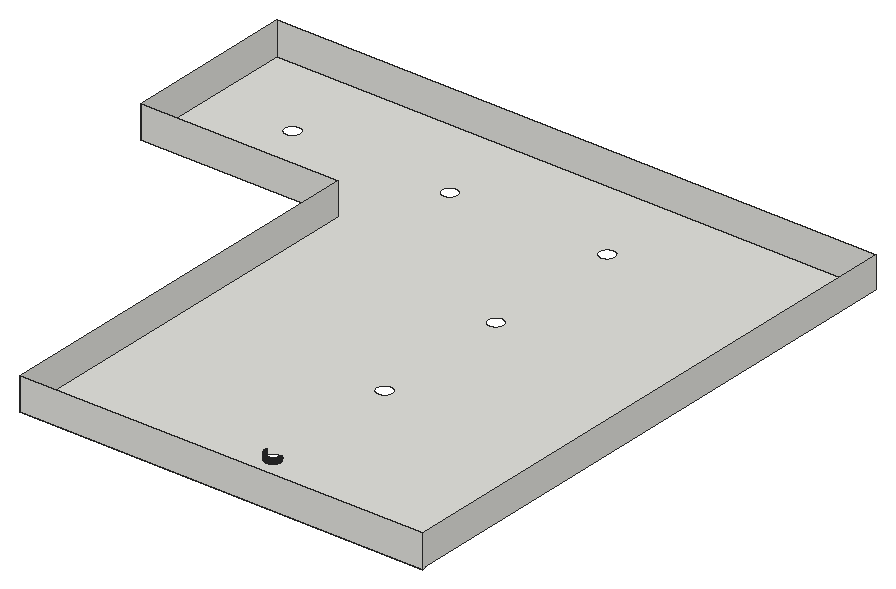
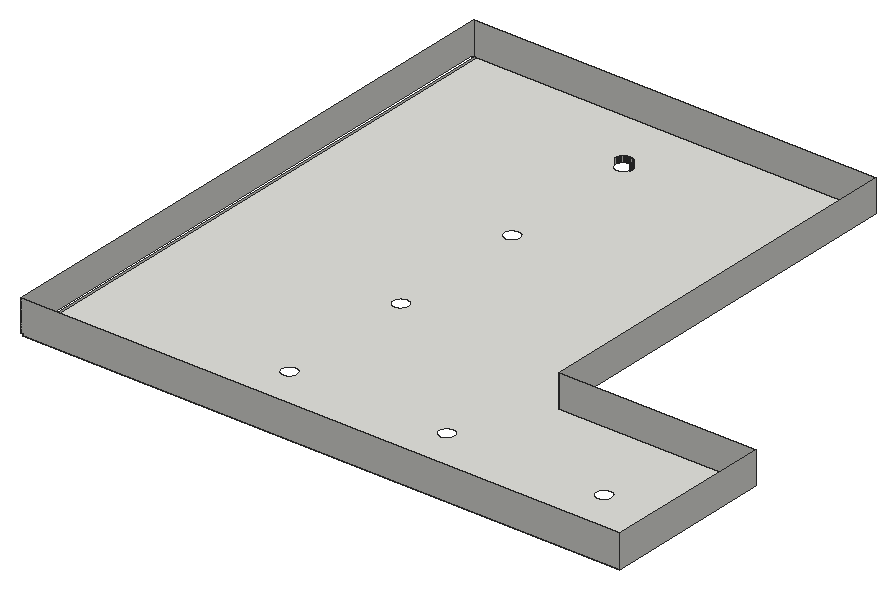
# SketchUp Ruby script. Lengths in inches.
U = 1.inch
M = Sketchup.active_model
def pt(a) = Geom::Point3d.new(a.map { |v| v * U })
def face(e, loops, mat)
  f = e.add_face(loops[0].map { |a| pt(a) })
  loops[1..].each { |l| e.add_face(l.map { |a| pt(a) }).erase! }
  f.material = f.back_material = mat if mat
  f
end
# faces: each face lists its corners as indices into pts; further lists are holes
def faces(e, pts, list, mat = nil) = list.each { |f| face(e, (f[0].is_a?(Array) ? f : [f]).map { |l| l.map { |i| pts[i] } }, mat) }
# xy, xz, yz: faces in a plane at the given z, y or x. An outline is a flat list of corners, or four numbers for a rectangle; further outlines are holes
def ring(l) = l.size == 4 ? [[l[0], l[1]], [l[2], l[1]], [l[2], l[3]], [l[0], l[3]]] : l.each_slice(2).to_a
def flat(e, list, mat, &to3) = list.each { |f| face(e, (f[0].is_a?(Array) ? f : [f]).map { |l| ring(l).map { |u, v| to3.(u, v) } }, mat) }
def xy(e, z, list, mat = nil) = flat(e, list, mat) { |x, y| [x, y, z] }
def xz(e, y, list, mat = nil) = flat(e, list, mat) { |x, z| [x, y, z] }
def yz(e, x, list, mat = nil) = flat(e, list, mat) { |y, z| [x, y, z] }
def lines(e, pts, list) = list.each { |a, b| e.add_line(pt(pts[a]), pt(pts[b])) }
# prism: a flat outline (further loops are holes) pulled along v
def prism(e, loops, v, mat = nil)
  f = face(e, loops, mat); d = Geom::Vector3d.new(v.map { |x| x * U })
  f.pushpull(f.normal.samedirection?(d) ? d.length : -d.length)
end
def box(e, o, s, mat = nil) = prism(e, [[o, [o[0] + s[0], o[1], o[2]], [o[0] + s[0], o[1] + s[1], o[2]], [o[0], o[1] + s[1], o[2]]]], [0, 0, s[2]], mat)
def at(x, y, z, deg = 0) = Geom::Transformation.translation(pt([x, y, z])) * Geom::Transformation.rotation(ORIGIN, Z_AXIS, deg.degrees)
def axes(o, x, y, z) = Geom::Transformation.new([*x, 0, *y, 0, *z, 0, *pt(o).to_a, 1])
def part(name) = M.definitions.add(name)
# library, detail: a bought-in or finely detailed component or shape, given as its bounding box
def library(name, o, s) = part(name).tap { |d| box(d.entities, o, s) }
def detail(e, o, s) = box(e.add_group.entities, o, s)
def put(e, d, t, mat = nil) = e.add_instance(d, t).tap { |i| i.material = mat if mat }
def group(e, t, mat = nil) = e.add_group.tap { |g| g.transformation = t; g.material = mat if mat }.entities
root = M.entities
xy(root,108,[[[82,0,82,147,9,147,9,210,230,210,230,1,231,1,231,0],[156.34,175.5,156.66,175.5,156.74,175.51,156.8125,175.52,156.89,175.53,157.05,175.55,157.125,175.57,157.2,175.58,157.28,175.6,157.35,175.625,157.43,175.65,157.5,175.67,157.58,175.7,157.79,175.79,157.86,175.83,157.93,175.86,158.07,175.94,158.13,175.98,158.2,176.03,158.26,176.07,158.33,176.12,158.57,176.32,158.62,176.38,158.68,176.43,158.88,176.67,158.93,176.74,158.97,176.8,159.02,176.87,159.06,176.93,159.14,177.07,159.17,177.14,159.21,177.21,159.3,177.42,159.33,177.5,159.35,177.57,159.375,177.65,159.4,177.72,159.42,177.8,159.43,177.875,159.45,177.95,159.47,178.11,159.48,178.1875,159.49,178.26,159.5,178.34,159.5,178.66,159.49,178.74,159.48,178.8125,159.47,178.89,159.45,179.05,159.43,179.125,159.42,179.2,159.4,179.28,159.375,179.35,159.35,179.43,159.33,179.5,159.3,179.58,159.21,179.79,159.17,179.86,159.14,179.93,159.06,180.07,159.02,180.13,158.97,180.2,158.93,180.26,158.88,180.33,158.68,180.57,158.62,180.62,158.57,180.68,158.33,180.88,158.26,180.93,158.2,180.97,158.13,181.02,158.07,181.06,157.93,181.14,157.86,181.17,157.79,181.21,157.58,181.3,157.5,181.33,157.43,181.35,157.35,181.375,157.28,181.4,157.2,181.42,157.125,181.43,157.05,181.45,156.89,181.47,156.8125,181.48,156.74,181.49,156.66,181.5,156.34,181.5,156.26,181.49,156.1875,181.48,156.11,181.47,155.95,181.45,155.875,181.43,155.8,181.42,155.72,181.4,155.65,181.375,155.57,181.35,155.5,181.33,155.42,181.3,155.21,181.21,155.14,181.17,155.07,181.14,154.93,181.06,154.87,181.02,154.8,180.97,154.74,180.93,154.67,180.88,154.43,180.68,154.38,180.62,154.32,180.57,154.12,180.33,154.07,180.26,154.03,180.2,153.98,180.13,153.94,180.07,153.86,179.93,153.83,179.86,153.79,179.79,153.7,179.58,153.67,179.5,153.65,179.43,153.625,179.35,153.6,179.28,153.58,179.2,153.57,179.125,153.55,179.05,153.53,178.89,153.52,178.8125,153.51,178.74,153.5,178.66,153.5,178.34,153.51,178.26,153.52,178.1875,153.53,178.11,153.55,177.95,153.57,177.875,153.58,177.8,153.6,177.72,153.625,177.65,153.65,177.57,153.67,177.5,153.7,177.42,153.79,177.21,153.83,177.14,153.86,177.07,153.94,176.93,153.98,176.87,154.03,176.8,154.07,176.74,154.12,176.67,154.32,176.43,154.38,176.38,154.43,176.32,154.67,176.12,154.74,176.07,154.8,176.03,154.87,175.98,154.93,175.94,155.07,175.86,155.14,175.83,155.21,175.79,155.42,175.7,155.5,175.67,155.57,175.65,155.65,175.625,155.72,175.6,155.8,175.58,155.875,175.57,155.95,175.55,156.11,175.53,156.1875,175.52,156.26,175.51],[156.34,124,156.66,124,156.74,124.01,156.8125,124.02,156.89,124.03,157.05,124.05,157.125,124.07,157.2,124.08,157.28,124.1,157.35,124.125,157.43,124.15,157.5,124.17,157.58,124.2,157.79,124.29,157.86,124.33,157.93,124.36,158.07,124.44,158.13,124.48,158.2,124.53,158.26,124.57,158.33,124.62,158.57,124.82,158.62,124.88,158.68,124.93,158.88,125.17,158.93,125.24,158.97,125.3,159.02,125.37,159.06,125.43,159.14,125.57,159.17,125.64,159.21,125.71,159.3,125.92,159.33,126,159.35,126.07,159.375,126.15,159.4,126.22,159.42,126.3,159.43,126.375,159.45,126.45,159.47,126.61,159.48,126.6875,159.49,126.76,159.5,126.84,159.5,127.16,159.49,127.24,159.48,127.3125,159.47,127.39,159.45,127.55,159.43,127.625,159.42,127.7,159.4,127.78,159.375,127.85,159.35,127.93,159.33,128,159.3,128.08,159.21,128.29,159.17,128.36,159.14,128.43,159.06,128.57,159.02,128.63,158.97,128.7,158.93,128.76,158.88,128.83,158.68,129.07,158.62,129.12,158.57,129.18,158.33,129.38,158.26,129.43,158.2,129.47,158.13,129.52,158.07,129.56,157.93,129.64,157.86,129.67,157.79,129.71,157.58,129.8,157.5,129.83,157.43,129.85,157.35,129.875,157.28,129.9,157.2,129.92,157.125,129.93,157.05,129.95,156.89,129.97,156.8125,129.98,156.74,129.99,156.66,130,156.34,130,156.26,129.99,156.1875,129.98,156.11,129.97,155.95,129.95,155.875,129.93,155.8,129.92,155.72,129.9,155.65,129.875,155.57,129.85,155.5,129.83,155.42,129.8,155.21,129.71,155.14,129.67,155.07,129.64,154.93,129.56,154.87,129.52,154.8,129.47,154.74,129.43,154.67,129.38,154.43,129.18,154.38,129.12,154.32,129.07,154.12,128.83,154.07,128.76,154.03,128.7,153.98,128.63,153.94,128.57,153.86,128.43,153.83,128.36,153.79,128.29,153.7,128.08,153.67,128,153.65,127.93,153.625,127.85,153.6,127.78,153.58,127.7,153.57,127.625,153.55,127.55,153.53,127.39,153.52,127.3125,153.51,127.24,153.5,127.16,153.5,126.84,153.51,126.76,153.52,126.6875,153.53,126.61,153.55,126.45,153.57,126.375,153.58,126.3,153.6,126.22,153.625,126.15,153.65,126.07,153.67,126,153.7,125.92,153.79,125.71,153.83,125.64,153.86,125.57,153.94,125.43,153.98,125.37,154.03,125.3,154.07,125.24,154.12,125.17,154.32,124.93,154.38,124.88,154.43,124.82,154.67,124.62,154.74,124.57,154.8,124.53,154.87,124.48,154.93,124.44,155.07,124.36,155.14,124.33,155.21,124.29,155.42,124.2,155.5,124.17,155.57,124.15,155.65,124.125,155.72,124.1,155.8,124.08,155.875,124.07,155.95,124.05,156.11,124.03,156.1875,124.02,156.26,124.01],[156.34,72.5,156.66,72.5,156.74,72.51,156.8125,72.52,156.89,72.53,157.05,72.55,157.125,72.57,157.2,72.58,157.28,72.6,157.35,72.625,157.43,72.65,157.5,72.67,157.58,72.7,157.79,72.79,157.86,72.83,157.93,72.86,158.07,72.94,158.13,72.98,158.2,73.03,158.26,73.07,158.33,73.12,158.57,73.32,158.62,73.38,158.68,73.43,158.88,73.67,158.93,73.74,158.97,73.8,159.02,73.87,159.06,73.93,159.14,74.07,159.17,74.14,159.21,74.21,159.3,74.42,159.33,74.5,159.35,74.57,159.375,74.65,159.4,74.72,159.42,74.8,159.43,74.875,159.45,74.95,159.47,75.11,159.48,75.1875,159.49,75.26,159.5,75.34,159.5,75.66,159.49,75.74,159.48,75.8125,159.47,75.89,159.45,76.05,159.43,76.125,159.42,76.2,159.4,76.28,159.375,76.35,159.35,76.43,159.33,76.5,159.3,76.58,159.21,76.79,159.17,76.86,159.14,76.93,159.06,77.07,159.02,77.13,158.97,77.2,158.93,77.26,158.88,77.33,158.68,77.57,158.62,77.62,158.57,77.68,158.33,77.88,158.26,77.93,158.2,77.97,158.13,78.02,158.07,78.06,157.93,78.14,157.86,78.17,157.79,78.21,157.58,78.3,157.5,78.33,157.43,78.35,157.35,78.375,157.28,78.4,157.2,78.42,157.125,78.43,157.05,78.45,156.89,78.47,156.8125,78.48,156.74,78.49,156.66,78.5,156.34,78.5,156.26,78.49,156.1875,78.48,156.11,78.47,155.95,78.45,155.875,78.43,155.8,78.42,155.72,78.4,155.65,78.375,155.57,78.35,155.5,78.33,155.42,78.3,155.21,78.21,155.14,78.17,155.07,78.14,154.93,78.06,154.87,78.02,154.8,77.97,154.74,77.93,154.67,77.88,154.43,77.68,154.38,77.62,154.32,77.57,154.12,77.33,154.07,77.26,154.03,77.2,153.98,77.13,153.94,77.07,153.86,76.93,153.83,76.86,153.79,76.79,153.7,76.58,153.67,76.5,153.65,76.43,153.625,76.35,153.6,76.28,153.58,76.2,153.57,76.125,153.55,76.05,153.53,75.89,153.52,75.8125,153.51,75.74,153.5,75.66,153.5,75.34,153.51,75.26,153.52,75.1875,153.53,75.11,153.55,74.95,153.57,74.875,153.58,74.8,153.6,74.72,153.625,74.65,153.65,74.57,153.67,74.5,153.7,74.42,153.79,74.21,153.83,74.14,153.86,74.07,153.94,73.93,153.98,73.87,154.03,73.8,154.07,73.74,154.12,73.67,154.32,73.43,154.38,73.38,154.43,73.32,154.67,73.12,154.74,73.07,154.8,73.03,154.87,72.98,154.93,72.94,155.07,72.86,155.14,72.83,155.21,72.79,155.42,72.7,155.5,72.67,155.57,72.65,155.65,72.625,155.72,72.6,155.8,72.58,155.875,72.57,155.95,72.55,156.11,72.53,156.1875,72.52,156.26,72.51],[156.34,21,156.66,21,156.74,21.01,156.8125,21.02,156.89,21.03,157.05,21.05,157.125,21.07,157.2,21.08,157.28,21.1,157.35,21.125,157.43,21.15,157.5,21.17,157.58,21.2,157.79,21.29,157.86,21.33,157.93,21.36,158.07,21.44,158.13,21.48,158.2,21.53,158.26,21.57,158.33,21.62,158.57,21.82,158.62,21.88,158.68,21.93,158.88,22.17,158.93,22.24,158.97,22.3,159.02,22.37,159.06,22.43,159.14,22.57,159.17,22.64,159.21,22.71,159.3,22.92,159.33,23,159.35,23.07,159.375,23.15,159.4,23.22,159.42,23.3,159.43,23.375,159.45,23.45,159.47,23.61,159.48,23.6875,159.49,23.76,159.5,23.84,159.5,24.16,159.49,24.24,159.48,24.3125,159.47,24.39,159.45,24.55,159.43,24.625,159.42,24.7,159.4,24.78,159.375,24.85,159.35,24.93,159.33,25,159.3,25.08,159.21,25.29,159.17,25.36,159.14,25.43,159.06,25.57,159.02,25.63,158.97,25.7,158.93,25.76,158.88,25.83,158.68,26.07,158.62,26.12,158.57,26.18,158.33,26.38,158.26,26.43,158.2,26.47,158.13,26.52,158.07,26.56,157.93,26.64,157.86,26.67,157.79,26.71,157.58,26.8,157.5,26.83,157.43,26.85,157.35,26.875,157.28,26.9,157.2,26.92,157.125,26.93,157.05,26.95,156.89,26.97,156.8125,26.98,156.74,26.99,156.66,27,156.34,27,156.26,26.99,156.1875,26.98,156.11,26.97,155.95,26.95,155.875,26.93,155.8,26.92,155.72,26.9,155.65,26.875,155.57,26.85,155.5,26.83,155.42,26.8,155.21,26.71,155.14,26.67,155.07,26.64,154.93,26.56,154.87,26.52,154.8,26.47,154.74,26.43,154.67,26.38,154.43,26.18,154.38,26.12,154.32,26.07,154.12,25.83,154.07,25.76,154.03,25.7,153.98,25.63,153.94,25.57,153.86,25.43,153.83,25.36,153.79,25.29,153.7,25.08,153.67,25,153.65,24.93,153.625,24.85,153.6,24.78,153.58,24.7,153.57,24.625,153.55,24.55,153.53,24.39,153.52,24.3125,153.51,24.24,153.5,24.16,153.5,23.84,153.51,23.76,153.52,23.6875,153.53,23.61,153.55,23.45,153.57,23.375,153.58,23.3,153.6,23.22,153.625,23.15,153.65,23.07,153.67,23,153.7,22.92,153.79,22.71,153.83,22.64,153.86,22.57,153.94,22.43,153.98,22.37,154.03,22.3,154.07,22.24,154.12,22.17,154.32,21.93,154.38,21.88,154.43,21.82,154.67,21.62,154.74,21.57,154.8,21.53,154.87,21.48,154.93,21.44,155.07,21.36,155.14,21.33,155.21,21.29,155.42,21.2,155.5,21.17,155.57,21.15,155.65,21.125,155.72,21.1,155.8,21.08,155.875,21.07,155.95,21.05,156.11,21.03,156.1875,21.02,156.26,21.01],[98.09,175.5,98.41,175.5,98.49,175.51,98.5625,175.52,98.64,175.53,98.8,175.55,98.875,175.57,98.95,175.58,99.03,175.6,99.1,175.625,99.18,175.65,99.25,175.67,99.33,175.7,99.54,175.79,99.61,175.83,99.68,175.86,99.82,175.94,99.88,175.98,99.95,176.03,100.01,176.07,100.08,176.12,100.32,176.32,100.37,176.38,100.43,176.43,100.63,176.67,100.68,176.74,100.72,176.8,100.77,176.87,100.81,176.93,100.89,177.07,100.92,177.14,100.96,177.21,101.05,177.42,101.08,177.5,101.1,177.57,101.125,177.65,101.15,177.72,101.17,177.8,101.18,177.875,101.2,177.95,101.22,178.11,101.23,178.1875,101.24,178.26,101.25,178.34,101.25,178.66,101.24,178.74,101.23,178.8125,101.22,178.89,101.2,179.05,101.18,179.125,101.17,179.2,101.15,179.28,101.125,179.35,101.1,179.43,101.08,179.5,101.05,179.58,100.96,179.79,100.92,179.86,100.89,179.93,100.81,180.07,100.77,180.13,100.72,180.2,100.68,180.26,100.63,180.33,100.43,180.57,100.37,180.62,100.32,180.68,100.08,180.88,100.01,180.93,99.95,180.97,99.88,181.02,99.82,181.06,99.68,181.14,99.61,181.17,99.54,181.21,99.33,181.3,99.25,181.33,99.18,181.35,99.1,181.375,99.03,181.4,98.95,181.42,98.875,181.43,98.8,181.45,98.64,181.47,98.5625,181.48,98.49,181.49,98.41,181.5,98.09,181.5,98.01,181.49,97.9375,181.48,97.86,181.47,97.7,181.45,97.625,181.43,97.55,181.42,97.47,181.4,97.4,181.375,97.32,181.35,97.25,181.33,97.17,181.3,96.96,181.21,96.89,181.17,96.82,181.14,96.68,181.06,96.62,181.02,96.55,180.97,96.49,180.93,96.42,180.88,96.18,180.68,96.13,180.62,96.07,180.57,95.87,180.33,95.82,180.26,95.78,180.2,95.73,180.13,95.69,180.07,95.61,179.93,95.58,179.86,95.54,179.79,95.45,179.58,95.42,179.5,95.4,179.43,95.375,179.35,95.35,179.28,95.33,179.2,95.32,179.125,95.3,179.05,95.28,178.89,95.27,178.8125,95.26,178.74,95.25,178.66,95.25,178.34,95.26,178.26,95.27,178.1875,95.28,178.11,95.3,177.95,95.32,177.875,95.33,177.8,95.35,177.72,95.375,177.65,95.4,177.57,95.42,177.5,95.45,177.42,95.54,177.21,95.58,177.14,95.61,177.07,95.69,176.93,95.73,176.87,95.78,176.8,95.82,176.74,95.87,176.67,96.07,176.43,96.13,176.38,96.18,176.32,96.42,176.12,96.49,176.07,96.55,176.03,96.62,175.98,96.68,175.94,96.82,175.86,96.89,175.83,96.96,175.79,97.17,175.7,97.25,175.67,97.32,175.65,97.4,175.625,97.47,175.6,97.55,175.58,97.625,175.57,97.7,175.55,97.86,175.53,97.9375,175.52,98.01,175.51],[39.84,175.5,40.16,175.5,40.24,175.51,40.3125,175.52,40.39,175.53,40.55,175.55,40.625,175.57,40.7,175.58,40.78,175.6,40.85,175.625,40.93,175.65,41,175.67,41.08,175.7,41.29,175.79,41.36,175.83,41.43,175.86,41.57,175.94,41.63,175.98,41.7,176.03,41.76,176.07,41.83,176.12,42.07,176.32,42.12,176.38,42.18,176.43,42.38,176.67,42.43,176.74,42.47,176.8,42.52,176.87,42.56,176.93,42.64,177.07,42.67,177.14,42.71,177.21,42.8,177.42,42.83,177.5,42.85,177.57,42.875,177.65,42.9,177.72,42.92,177.8,42.93,177.875,42.95,177.95,42.97,178.11,42.98,178.1875,42.99,178.26,43,178.34,43,178.66,42.99,178.74,42.98,178.8125,42.97,178.89,42.95,179.05,42.93,179.125,42.92,179.2,42.9,179.28,42.875,179.35,42.85,179.43,42.83,179.5,42.8,179.58,42.71,179.79,42.67,179.86,42.64,179.93,42.56,180.07,42.52,180.13,42.47,180.2,42.43,180.26,42.38,180.33,42.18,180.57,42.12,180.62,42.07,180.68,41.83,180.88,41.76,180.93,41.7,180.97,41.63,181.02,41.57,181.06,41.43,181.14,41.36,181.17,41.29,181.21,41.08,181.3,41,181.33,40.93,181.35,40.85,181.375,40.78,181.4,40.7,181.42,40.625,181.43,40.55,181.45,40.39,181.47,40.3125,181.48,40.24,181.49,40.16,181.5,39.84,181.5,39.76,181.49,39.6875,181.48,39.61,181.47,39.45,181.45,39.375,181.43,39.3,181.42,39.22,181.4,39.15,181.375,39.07,181.35,39,181.33,38.92,181.3,38.71,181.21,38.64,181.17,38.57,181.14,38.43,181.06,38.37,181.02,38.3,180.97,38.24,180.93,38.17,180.88,37.93,180.68,37.88,180.62,37.82,180.57,37.62,180.33,37.57,180.26,37.53,180.2,37.48,180.13,37.44,180.07,37.36,179.93,37.33,179.86,37.29,179.79,37.2,179.58,37.17,179.5,37.15,179.43,37.125,179.35,37.1,179.28,37.08,179.2,37.07,179.125,37.05,179.05,37.03,178.89,37.02,178.8125,37.01,178.74,37,178.66,37,178.34,37.01,178.26,37.02,178.1875,37.03,178.11,37.05,177.95,37.07,177.875,37.08,177.8,37.1,177.72,37.125,177.65,37.15,177.57,37.17,177.5,37.2,177.42,37.29,177.21,37.33,177.14,37.36,177.07,37.44,176.93,37.48,176.87,37.53,176.8,37.57,176.74,37.62,176.67,37.82,176.43,37.88,176.38,37.93,176.32,38.17,176.12,38.24,176.07,38.3,176.03,38.37,175.98,38.43,175.94,38.57,175.86,38.64,175.83,38.71,175.79,38.92,175.7,39,175.67,39.07,175.65,39.15,175.625,39.22,175.6,39.3,175.58,39.375,175.57,39.45,175.55,39.61,175.53,39.6875,175.52,39.76,175.51]]])
xz(root,0,[[82,108,231,120]])
xz(root,1,[[230,108,231,108.5]])
xz(root,21,[[156.34,108,156.42,110],[156.42,108,156.5,110],[156.5,108,156.58,110],[156.58,108,156.66,110]])
xz(root,147,[[9,108,82,120]])
xz(root,210,[[9,108,9,120,231,120,231,108.5,230,108.5,230,108]])
yz(root,9,[[147,108,210,120]])
yz(root,82,[[0,108,147,120]])
yz(root,153.5,[[23.84,108,23.92,110],[23.92,108,24,110],[24,108,24.08,110],[24.08,108,24.16,110]])
yz(root,159.5,[[23.84,108,23.92,110],[23.92,108,24,110]])
yz(root,230,[[1,108,210,108.5]])
yz(root,231,[[0,108,1,108,1,108.5,210,108.5,210,120,0,120]])
p = [[156.11,21.03,108],[156.03,21.04,108],[156.03,21.04,110],[156.11,21.03,110],[155.95,21.05,108],[155.95,21.05,110],
  [156.1875,21.02,108],[156.1875,21.02,110],[156.26,21.01,108],[156.26,21.01,110],[156.34,21,108],[156.34,21,110],
  [156.8125,21.02,108],[156.74,21.01,108],[156.74,21.01,110],[156.8125,21.02,110],[156.66,21,108],[156.66,21,110],
  [156.89,21.03,108],[156.89,21.03,110],[156.97,21.04,108],[156.97,21.04,110],[157.05,21.05,108],[157.05,21.05,110],
  [155.57,21.15,108],[155.5,21.17,108],[155.5,21.17,110],[155.57,21.15,110],[155.72,21.1,108],[155.65,21.125,108],
  [155.65,21.125,110],[155.72,21.1,110],[155.8,21.08,108],[155.8,21.08,110],[155.875,21.07,108],[155.875,21.07,110],
  [157.125,21.07,108],[157.125,21.07,110],[157.2,21.08,108],[157.2,21.08,110],[157.28,21.1,108],[157.28,21.1,110],
  [157.35,21.125,108],[157.35,21.125,110],[157.5,21.17,108],[157.43,21.15,108],[157.43,21.15,110],[157.5,21.17,110],
  [155.35,21.23,108],[155.28,21.26,108],[155.28,21.26,110],[155.35,21.23,110],[155.42,21.2,108],[155.42,21.2,110],
  [157.58,21.2,108],[157.58,21.2,110],[157.72,21.26,108],[157.65,21.23,108],[157.65,21.23,110],[157.72,21.26,110],
  [155.21,21.29,108],[155.14,21.33,108],[155.14,21.33,110],[155.21,21.29,110],[155.07,21.36,108],[155.07,21.36,110],
  [157.79,21.29,108],[157.79,21.29,110],[157.86,21.33,108],[157.86,21.33,110],[157.93,21.36,108],[157.93,21.36,110],
  [155,21.4,108],[154.93,21.44,108],[154.93,21.44,110],[155,21.4,110],[154.87,21.48,108],[154.87,21.48,110],
  [158,21.4,108],[158,21.4,110],[158.07,21.44,108],[158.07,21.44,110],[158.13,21.48,108],[158.13,21.48,110],
  [154.8,21.53,108],[154.74,21.57,108],[154.74,21.57,110],[154.8,21.53,110],[158.2,21.53,108],[158.2,21.53,110],
  [158.26,21.57,108],[158.26,21.57,110],[154.67,21.62,108],[154.61,21.67,108],[154.61,21.67,110],[154.67,21.62,110],
  [158.39,21.67,108],[158.33,21.62,108],[158.33,21.62,110],[158.39,21.67,110],[154.55,21.72,108],[154.49,21.77,108],
  [154.49,21.77,110],[154.55,21.72,110],[158.51,21.77,108],[158.45,21.72,108],[158.45,21.72,110],[158.51,21.77,110],
  [154.43,21.82,108],[154.43,21.82,110],[154.38,21.88,108],[154.38,21.88,110],[158.57,21.82,108],[158.57,21.82,110],
  [158.62,21.88,108],[158.62,21.88,110],[154.32,21.93,108],[154.32,21.93,110],[154.27,21.99,108],[154.27,21.99,110],
  [158.68,21.93,108],[158.68,21.93,110],[158.73,21.99,108],[158.73,21.99,110],[154.22,22.05,108],[154.22,22.05,110],
  [158.78,22.05,108],[158.78,22.05,110],[154.17,22.11,108],[154.12,22.17,108],[154.12,22.17,110],[154.17,22.11,110],
  [158.88,22.17,108],[158.83,22.11,108],[158.83,22.11,110],[158.88,22.17,110],[154.07,22.24,108],[154.03,22.3,108],
  [154.03,22.3,110],[154.07,22.24,110],[158.97,22.3,108],[158.93,22.24,108],[158.93,22.24,110],[158.97,22.3,110],
  [153.98,22.37,108],[153.98,22.37,110],[159.02,22.37,108],[159.02,22.37,110],[153.94,22.43,108],[153.94,22.43,110],
  [153.9,22.5,108],[153.9,22.5,110],[159.06,22.43,108],[159.06,22.43,110],[159.1,22.5,108],[159.1,22.5,110],
  [153.86,22.57,108],[153.86,22.57,110],[159.14,22.57,108],[159.14,22.57,110],[153.83,22.64,108],[153.83,22.64,110],
  [153.79,22.71,108],[153.79,22.71,110],[159.17,22.64,108],[159.17,22.64,110],[159.21,22.71,108],[159.21,22.71,110],
  [153.76,22.78,108],[153.76,22.78,110],[159.24,22.78,108],[159.24,22.78,110],[153.73,22.85,108],[153.73,22.85,110],
  [159.27,22.85,108],[159.27,22.85,110],[153.7,22.92,108],[153.7,22.92,110],[153.67,23,108],[153.67,23,110],
  [159.33,23,108],[159.3,22.92,108],[159.3,22.92,110],[159.33,23,110],[153.65,23.07,108],[153.65,23.07,110],
  [159.35,23.07,108],[159.35,23.07,110],[153.625,23.15,108],[153.625,23.15,110],[153.6,23.22,108],[153.6,23.22,110],
  [159.4,23.22,108],[159.375,23.15,108],[159.375,23.15,110],[159.4,23.22,110],[153.58,23.3,108],[153.58,23.3,110],
  [159.42,23.3,108],[159.42,23.3,110],[153.57,23.375,108],[153.57,23.375,110],[159.43,23.375,108],[159.43,23.375,110],
  [153.55,23.45,108],[153.55,23.45,110],[159.45,23.45,108],[159.45,23.45,110],[153.54,23.53,108],[153.54,23.53,110],
  [153.53,23.61,108],[153.53,23.61,110],[159.46,23.53,108],[159.46,23.53,110],[159.47,23.61,108],[159.47,23.61,110],
  [153.52,23.6875,108],[153.52,23.6875,110],[159.48,23.6875,108],[159.48,23.6875,110],[153.51,23.76,108],[153.51,23.76,110],
  [159.49,23.76,108],[159.49,23.76,110],[153.5,23.84,108],[153.5,23.84,110],[159.5,23.84,108],[159.5,23.84,110],
  [153.5,24.16,108],[153.51,24.24,108],[153.51,24.24,110],[153.5,24.16,110],[153.52,24.3125,108],[153.52,24.3125,110],
  [153.53,24.39,108],[153.53,24.39,110],[153.54,24.47,108],[153.54,24.47,110],[153.55,24.55,108],[153.55,24.55,110]]
faces(root,p,[[0,1,2,3],[1,4,5,2],[6,0,3,7],[8,6,7,9],[10,8,9,11],[12,13,14,15],[13,16,17,14],[18,12,15,19],
  [20,18,19,21],[22,20,21,23],[24,25,26,27],[28,29,30,31],[29,24,27,30],[32,28,31,33],[34,32,33,35],[4,34,35,5],
  [36,22,23,37],[38,36,37,39],[40,38,39,41],[42,40,41,43],[44,45,46,47],[45,42,43,46],[48,49,50,51],[25,52,53,26],
  [52,48,51,53],[54,44,47,55],[56,57,58,59],[57,54,55,58],[60,61,62,63],[61,64,65,62],[49,60,63,50],[66,56,59,67],
  [68,66,67,69],[70,68,69,71],[72,73,74,75],[73,76,77,74],[64,72,75,65],[78,70,71,79],[80,78,79,81],[82,80,81,83],
  [84,85,86,87],[76,84,87,77],[88,82,83,89],[90,88,89,91],[92,93,94,95],[85,92,95,86],[96,97,98,99],[97,90,91,98],
  [100,101,102,103],[93,100,103,94],[104,105,106,107],[105,96,99,106],[101,108,109,102],[108,110,111,109],[112,104,107,113],[114,112,113,115],
  [110,116,117,111],[116,118,119,117],[120,114,115,121],[122,120,121,123],[118,124,125,119],[126,122,123,127],[128,129,130,131],[124,128,131,125],
  [132,133,134,135],[133,126,127,134],[136,137,138,139],[129,136,139,130],[140,141,142,143],[141,132,135,142],[137,144,145,138],[146,140,143,147],
  [144,148,149,145],[148,150,151,149],[152,146,147,153],[154,152,153,155],[150,156,157,151],[158,154,155,159],[156,160,161,157],[160,162,163,161],
  [164,158,159,165],[166,164,165,167],[162,168,169,163],[170,166,167,171],[168,172,173,169],[174,170,171,175],[172,176,177,173],[176,178,179,177],
  [180,181,182,183],[181,174,175,182],[178,184,185,179],[186,180,183,187],[184,188,189,185],[188,190,191,189],[192,193,194,195],[193,186,187,194],
  [190,196,197,191],[198,192,195,199],[196,200,201,197],[202,198,199,203],[200,204,205,201],[206,202,203,207],[204,208,209,205],[208,210,211,209],
  [212,206,207,213],[214,212,213,215],[210,216,217,211],[218,214,215,219],[216,220,221,217],[222,218,219,223],[220,224,225,221],[226,222,223,227],
  [228,229,230,231],[229,232,233,230],[232,234,235,233],[234,236,237,235],[236,238,239,237]])
